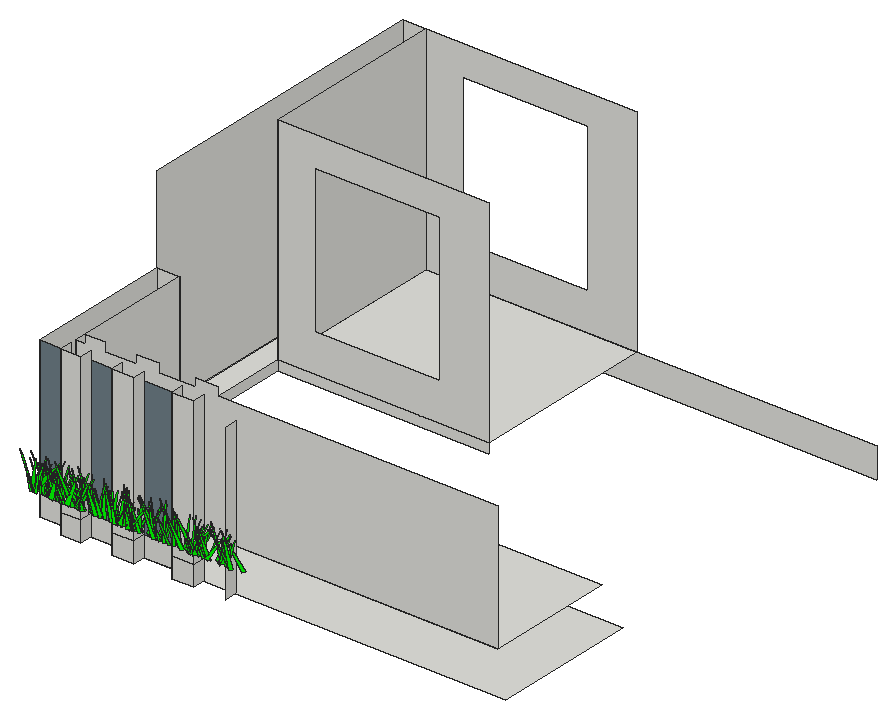
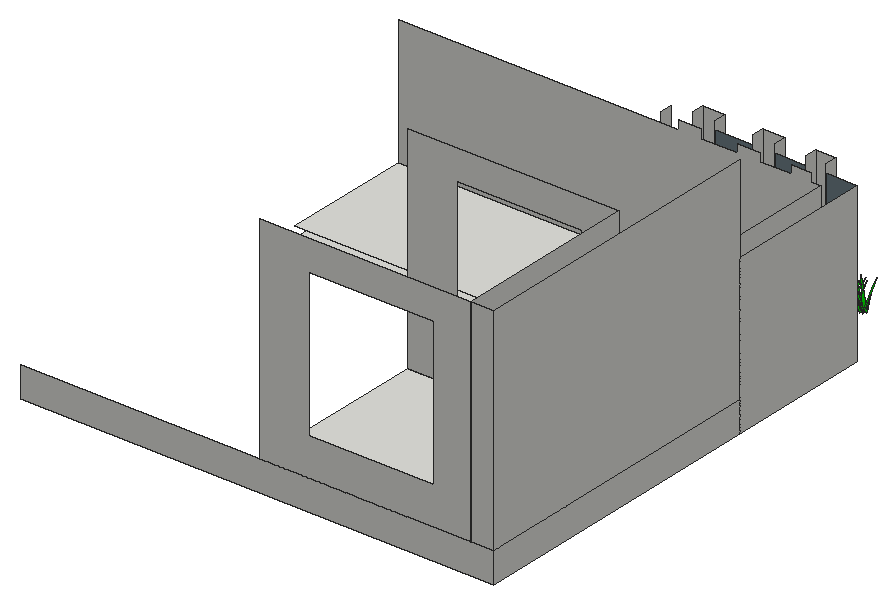
# SketchUp Ruby script. Lengths in inches.
U = 1.inch
M = Sketchup.active_model
def pt(a) = Geom::Point3d.new(a.map { |v| v * U })
def face(e, loops, mat)
  f = e.add_face(loops[0].map { |a| pt(a) })
  loops[1..].each { |l| e.add_face(l.map { |a| pt(a) }).erase! }
  f.material = f.back_material = mat if mat
  f
end
# faces: each face lists its corners as indices into pts; further lists are holes
def faces(e, pts, list, mat = nil) = list.each { |f| face(e, (f[0].is_a?(Array) ? f : [f]).map { |l| l.map { |i| pts[i] } }, mat) }
# xy, xz, yz: faces in a plane at the given z, y or x. An outline is a flat list of corners, or four numbers for a rectangle; further outlines are holes
def ring(l) = l.size == 4 ? [[l[0], l[1]], [l[2], l[1]], [l[2], l[3]], [l[0], l[3]]] : l.each_slice(2).to_a
def flat(e, list, mat, &to3) = list.each { |f| face(e, (f[0].is_a?(Array) ? f : [f]).map { |l| ring(l).map { |u, v| to3.(u, v) } }, mat) }
def xy(e, z, list, mat = nil) = flat(e, list, mat) { |x, y| [x, y, z] }
def xz(e, y, list, mat = nil) = flat(e, list, mat) { |x, z| [x, y, z] }
def yz(e, x, list, mat = nil) = flat(e, list, mat) { |y, z| [x, y, z] }
def lines(e, pts, list) = list.each { |a, b| e.add_line(pt(pts[a]), pt(pts[b])) }
# prism: a flat outline (further loops are holes) pulled along v
def prism(e, loops, v, mat = nil)
  f = face(e, loops, mat); d = Geom::Vector3d.new(v.map { |x| x * U })
  f.pushpull(f.normal.samedirection?(d) ? d.length : -d.length)
end
def box(e, o, s, mat = nil) = prism(e, [[o, [o[0] + s[0], o[1], o[2]], [o[0] + s[0], o[1] + s[1], o[2]], [o[0], o[1] + s[1], o[2]]]], [0, 0, s[2]], mat)
def at(x, y, z, deg = 0) = Geom::Transformation.translation(pt([x, y, z])) * Geom::Transformation.rotation(ORIGIN, Z_AXIS, deg.degrees)
def axes(o, x, y, z) = Geom::Transformation.new([*x, 0, *y, 0, *z, 0, *pt(o).to_a, 1])
def part(name) = M.definitions.add(name)
# library, detail: a bought-in or finely detailed component or shape, given as its bounding box
def library(name, o, s) = part(name).tap { |d| box(d.entities, o, s) }
def detail(e, o, s) = box(e.add_group.entities, o, s)
def put(e, d, t, mat = nil) = e.add_instance(d, t).tap { |i| i.material = mat if mat }
def group(e, t, mat = nil) = e.add_group.tap { |g| g.transformation = t; g.material = mat if mat }.entities
root = M.entities
M.materials.add("[0065_Lime]").color = [0, 255, 0]
M.materials.add("[0111_SlateGray]1").color = [112, 128, 136]
c1 = part("fur_instance\#9")
p = [[0.8125,0,1.79],[0.67,-0.02,1.48],[0,-0.11,0],[0,0.11,0]]
faces(c1.entities,p,[[0,1,2,3]])
xy(root,-11.8125,[[18.06,34.8125,25.54,39.75],[37.97,34.8125,46.56,39.75],[61.07,34.8125,69.9,39.75],[5.71,39.75,187.77,97.05]])
xy(root,0,[[14.21,46.62,179.21,97.05],[5.71,97.05,14.71,217.05],[14.71,144.8,96.96,217.05]])
xz(root,34.8125,[[18.06,-11.8125,25.54,-3.9375],[37.97,-11.8125,46.56,-3.9375],[61.07,-11.8125,69.9,-3.9375],[18.06,-3.9375,25.54,53.25],[37.97,-3.9375,46.56,53.25],
  [61.07,-3.9375,69.9,53.25]])
xz(root,39.75,[[5.71,-11.8125,18.06,-3.9375],[25.54,-11.8125,37.97,-3.9375],[46.56,-11.8125,61.07,-3.9375]])
xz(root,39.75,[[5.71,-3.9375,18.06,49.9375],[25.54,-3.9375,37.97,49.9375],[46.56,-3.9375,61.07,49.9375]],"[0111_SlateGray]1")
xz(root,46.62,[[14.21,0,14.21,49.9375,18.06,49.9375,18.06,53.25,25.54,53.25,25.54,49.9375,37.97,49.9375,37.97,53.25,46.56,53.25,46.56,49.9375,61.07,49.9375,61.07,53.25,69.9,53.25,69.9,49.9375,179.21,49.9375,179.21,0]])
xz(root,97.05,[[5.71,0,14.21,49.9375],[14.21,0,14.71,49.9375]])
xz(root,144.8,[[14.71,-3.9375,96.96,0],[[14.71,0,96.96,84],[29.05,14.85,77.86,72.35]]])
xz(root,217.05,[[5.71,-11.8125,190.59,0],[5.71,0,14.71,84],[[14.71,0,96.96,84],[29.05,14.85,77.86,72.35]]])
yz(root,5.71,[[39.75,-11.8125,97.05,49.9375],[97.05,-11.8125,217.05,0],[97.05,0,217.05,84]])
yz(root,14.21,[[46.62,0,97.05,49.9375]])
yz(root,14.71,[[97.05,-3.9375,144.8,0],[144.8,0,217.05,84]])
yz(root,18.06,[[34.8125,-11.8125,39.75,-3.9375],[34.8125,-3.9375,39.75,53.25]])
yz(root,25.54,[[34.8125,-11.8125,39.75,-3.9375],[34.8125,-3.9375,39.75,53.25]])
yz(root,37.97,[[34.8125,-11.8125,39.75,-3.9375],[34.8125,-3.9375,39.75,53.25]])
yz(root,46.56,[[34.8125,-11.8125,39.75,-3.9375],[34.8125,-3.9375,39.75,53.25]])
yz(root,61.07,[[34.8125,-11.8125,39.75,-3.9375],[34.8125,-3.9375,39.75,53.25]])
yz(root,69.9,[[34.8125,-11.8125,39.75,-3.9375],[34.8125,-3.9375,39.75,53.25]])
yz(root,82.49,[[34.4375,-11.6,39.75,48.65]])
put(root,c1,axes([41.71,32.27,1.48],[4.33195,0.11337,0.46115],[-0.98091,0.53224,1.7119],[-0.10114,-0.30594,3.14903]),"[0065_Lime]")
put(root,c1,axes([10.57,31.76,1.48],[-2.35976,0.59564,0.33042],[-4.03469,-0.33361,1.08708],[1.36172,0.04372,3.79354]),"[0065_Lime]")
put(root,c1,axes([70.67,32.28,1.48],[-4.46444,-0.02377,1.19402],[-0.39835,-0.61279,-1.39426],[1.42292,-0.24613,3.35594]),"[0065_Lime]")
put(root,c1,axes([62.18,32.23,1.48],[-2.3359,-0.64219,0.16019],[4.45315,-0.31213,1.03427],[-1.04619,0.10525,4.04472]),"[0065_Lime]")
put(root,c1,axes([21.09,32.11,1.48],[-5.80841,0.43314,0.64865],[-3.1839,-0.78871,-1.21559],[-0.01972,-0.238,5.20877]),"[0065_Lime]")
put(root,c1,axes([26.06,32.26,1.48],[-0.9862,-0.94635,1.83348],[6.30274,-0.264,-2.32294],[3.27302,0.22323,5.02564]),"[0065_Lime]")
put(root,c1,axes([56.34,31.98,1.48],[-6.05553,0.86304,0.84524],[-6.20995,-0.82043,-1.36562],[-0.48856,-0.26882,6.88155]),"[0065_Lime]")
put(root,c1,axes([8.38,32.48,1.48],[-2.48516,-1.08252,0.9385],[7.4377,-0.38033,-1.66901],[2.31515,0.05984,6.36929]),"[0065_Lime]")
put(root,c1,axes([77.67,32.27,1.48],[-0.79339,-0.86582,1.00223],[6.0769,-0.06133,1.40764],[-1.59867,0.19658,4.85336]),"[0065_Lime]")
put(root,c1,axes([86.75,31.84,1.48],[1.09455,1.06985,1.45468],[-7.35888,0.2268,-1.92578],[-2.64807,-0.18806,5.95294]),"[0065_Lime]")
put(root,c1,axes([46.66,32.18,1.48],[6.04785,0.54472,0.1694],[-3.68145,0.78754,2.10281],[1.23206,-0.32069,5.45175]),"[0065_Lime]")
put(root,c1,axes([48.66,31.79,1.48],[-4.51664,0.20117,0.17695],[-1.1949,-0.57433,1.69918],[0.81797,0.27182,3.45924]),"[0065_Lime]")
put(root,c1,axes([70.49,31.98,1.48],[-4.23495,-0.27981,1.01761],[2.33199,-0.5464,1.38671],[0.30344,0.29406,3.54499]),"[0065_Lime]")
put(root,c1,axes([14.39,32.3,1.48],[6.30222,-0.0403,1.72476],[-0.13396,0.91754,1.04218],[-2.1355,-0.17648,5.02467]),"[0065_Lime]")
put(root,c1,axes([42.49,32,1.48],[-7.14696,-0.2393,0.85014],[1.89816,-0.98349,1.28147],[0.62418,0.25076,5.83719]),"[0065_Lime]")
put(root,c1,axes([48.44,32.31,1.48],[2.36748,-1.00196,2.50606],[6.91986,0.47765,2.07402],[-3.52864,0.26446,5.74866]),"[0065_Lime]")
put(root,c1,axes([71.11,31.84,1.48],[5.66218,0.27971,0.02061],[-1.90106,0.76292,-1.39267],[-0.59075,0.22584,4.67916]),"[0065_Lime]")
put(root,c1,axes([67.18,32.29,1.48],[-6.69229,0.73041,1.14946],[-5.3124,-0.84253,-2.52432],[-0.89145,-0.4625,6.41386]),"[0065_Lime]")
put(root,c1,axes([19.09,32.36,1.48],[-5.70859,-0.071,1.72871],[0.02577,-0.83772,-1.0966],[2.18434,-0.17567,4.53078]),"[0065_Lime]")
put(root,c1,axes([26.21,32.26,1.48],[4.36818,-0.53106,0.3008],[3.76842,0.59646,-0.92106],[0.46817,0.15391,4.60727]),"[0065_Lime]")
put(root,c1,axes([72.5,32.2,1.48],[-0.48281,1.1024,3.21593],[-7.58977,0.22787,-3.37133],[-4.42435,-0.51119,5.43243]),"[0065_Lime]")
put(root,c1,axes([41.125,31.8,1.48],[-5.49042,0.65495,0.23007],[-4.49464,-0.75787,1.32632],[1.2661,0.14975,5.70613]),"[0065_Lime]")
put(root,c1,axes([8.66,32.14,1.48],[-1.90878,0.75502,1.27501],[-5.5526,-0.22615,-1.01257],[-0.70447,-0.26327,4.5263]),"[0065_Lime]")
put(root,c1,axes([50.56,32.2,1.48],[1.17059,-0.77851,2.66973],[5.86519,0.32241,1.4489],[-2.65841,0.36852,4.37225]),"[0065_Lime]")
put(root,c1,axes([86.15,32.24,1.48],[-5.07057,-0.84374,0.464],[5.57861,-0.61623,2.78679],[-2.29325,0.36654,5.75327]),"[0065_Lime]")
put(root,c1,axes([77,32.11,1.48],[3.53661,0.75197,0.25197],[-5.07953,0.45347,1.82348],[1.71241,-0.20791,4.88861]),"[0065_Lime]")
put(root,c1,axes([44.51,32.68,1.48],[8.0949,-0.61479,1.09274],[3.9513,1.13232,1.9803],[-2.30957,-0.21758,7.21798]),"[0065_Lime]")
put(root,c1,axes([16.28,31.9,1.48],[-2.53205,1.04954,1.22543],[-7.17157,-0.40363,1.7795],[2.57404,-0.09214,6.16333]),"[0065_Lime]")
put(root,c1,axes([24.72,32.36,1.48],[-4.40296,-1.10351,1.14391],[7.72191,-0.53272,2.44504],[-2.00544,0.37155,6.90312]),"[0065_Lime]")
put(root,c1,axes([27.31,32.54,1.48],[4.07818,-0.45781,0.32345],[3.06812,0.56339,1.12581],[-1.16594,-0.11876,4.09387]),"[0065_Lime]")
put(root,c1,axes([75.21,32.28,1.48],[-3.60754,0.42954,0.81253],[-3.21576,-0.47983,-0.94684],[-0.03047,-0.21549,3.72785]),"[0065_Lime]")
put(root,c1,axes([17.62,31.99,1.48],[-0.35804,0.98371,0.65762],[-6.75723,-0.01563,-1.65066],[-2.00056,-0.12326,5.45769]),"[0065_Lime]")
put(root,c1,axes([55.91,32.41,1.48],[-6.0947,0.51829,2.52587],[-4.41048,-0.88344,-0.96691],[1.94803,-0.37864,5.71342]),"[0065_Lime]")
put(root,c1,axes([9.09,32.45,1.48],[-8.66687,-0.05355,0.96269],[0.22891,-1.2198,-0.9103],[1.22212,-0.15131,6.9976]),"[0065_Lime]")
put(root,c1,axes([8.875,32.17,1.48],[-0.28933,0.60837,0.81065],[-4.26461,0.0013,-1.03981],[-1.2452,-0.14582,3.37285]),"[0065_Lime]")
put(root,c1,axes([35.36,32.43,1.48],[-0.19215,-0.90348,1.55262],[6.44119,0.04993,1.50107],[-1.86945,0.26491,5.01236]),"[0065_Lime]")
put(root,c1,axes([33.69,32.15,1.48],[-2.52802,1.00452,1.06299],[-7.10416,-0.30065,-1.65832],[-1.53077,-0.26367,5.94065]),"[0065_Lime]")
put(root,c1,axes([60.2,32.17,1.48],[8.32693,-0.25179,3.17868],[2.49423,1.25788,-0.98425],[-3.50156,0.29723,6.85802]),"[0065_Lime]")
put(root,c1,axes([58.74,31.97,1.48],[4.83244,0.23686,0.24352],[-1.38274,0.61427,-1.86589],[-1.00949,0.29248,3.72148]),"[0065_Lime]")
put(root,c1,axes([39.68,32.46,1.48],[-3.09092,-0.88211,2.44051],[6.39484,-0.54194,-1.20515],[2.74154,0.2696,5.56262]),"[0065_Lime]")
put(root,c1,axes([34.46,32.625,1.48],[-1.4279,-0.79185,0.65323],[5.46244,-0.22334,-1.17179],[1.60082,0.05578,4.58115]),"[0065_Lime]")
put(root,c1,axes([46.26,32.09,1.48],[2.60006,1.204,1.91417],[-8.5847,0.42928,-1.33269],[-2.29283,-0.24196,7.16045]),"[0065_Lime]")
put(root,c1,axes([70.95,31.94,1.48],[-7.33494,-0.2064,4.13991],[3.38747,-1.12188,2.09676],[4.07262,0.5614,5.71212]),"[0065_Lime]")
put(root,c1,axes([16.71,32.49,1.48],[5.57475,0.08869,0.24958],[-0.68368,0.76423,1.00416],[-0.15833,-0.17736,4.45169]),"[0065_Lime]")
put(root,c1,axes([20.8,32.42,1.48],[-2.29927,0.8627,1.81718],[-5.70084,-0.10237,-3.14405],[-3.19128,-0.43869,4.30721]),"[0065_Lime]")
put(root,c1,axes([84.91,32.6,1.48],[-2.69463,-0.69854,1.16109],[4.74631,-0.42384,-1.2565],[2.05501,0.06295,4.42454]),"[0065_Lime]")
put(root,c1,axes([11.92,32.18,1.48],[5.61368,0.50199,1.60112],[-3.37027,0.83591,-0.96357],[-2.29736,0.00032,5.32597]),"[0065_Lime]")
put(root,c1,axes([32.76,32.32,1.48],[-0.5471,-0.7816,2.4423],[6.04487,0.0591,1.52967],[-1.84771,0.42476,4.28122]),"[0065_Lime]")
put(root,c1,axes([22.58,31.98,1.48],[0.23893,1.12186,0.13379],[-7.74393,0.02691,1.58977],[1.94921,-0.03062,6.29952]),"[0065_Lime]")
put(root,c1,axes([73.35,32.4,1.48],[3.03492,-0.57134,1.24202],[4.34262,0.39472,-0.93657],[0.07407,0.26852,4.0194]),"[0065_Lime]")
put(root,c1,axes([9.59,32.37,1.48],[5.67515,-0.53055,1.42426],[4.10844,0.78065,-1.08694],[-0.66531,0.29505,5.43696]),"[0065_Lime]")
put(root,c1,axes([68.64,32.49,1.48],[5.8557,1.00358,0.75497],[-6.33522,0.63781,4.10122],[3.42561,-0.53597,6.29415]),"[0065_Lime]")
put(root,c1,axes([27.42,32.25,1.48],[-4.92428,0.00624,0.93904],[0.26433,-0.68529,1.06966],[1.12466,0.18838,3.86017]),"[0065_Lime]")
put(root,c1,axes([82.29,32.05,1.48],[-6.23404,0.04017,2.6623],[1.09701,-0.90438,2.15689],[3.09691,0.40122,4.59515]),"[0065_Lime]")
put(root,c1,axes([40.33,32.51,1.48],[6.78336,0.45066,1.50428],[-3.54224,0.94777,1.05405],[-1.07632,-0.27895,6.01159]),"[0065_Lime]")
put(root,c1,axes([50.05,32.87,1.48],[-2.20132,-1.06917,0.68439],[7.40379,-0.32862,-1.44655],[1.94578,0.04083,6.27845]),"[0065_Lime]")
put(root,c1,axes([81.4,32.5,1.48],[6.18641,0.52059,0.93806],[-3.87465,0.84509,1.19133],[-0.20672,-0.26033,5.7432]),"[0065_Lime]")
put(root,c1,axes([28.46,32.05,1.48],[3.11819,1.14666,1.5579],[-7.31821,0.51243,-2.94697],[-4.08676,-0.04272,6.46584]),"[0065_Lime]")
put(root,c1,axes([19.07,32.59,1.48],[5.55607,0.28488,0.41085],[-2.0865,0.74604,1.33504],[0.1088,-0.24082,4.6219]),"[0065_Lime]")
put(root,c1,axes([20.16,32.06,1.48],[7.88545,0.59374,0.96206],[-3.81,1.09606,-2.00481],[-2.1764,0.23247,6.99533]),"[0065_Lime]")
put(root,c1,axes([84.84,32.8,1.48],[0.39788,-0.77961,0.32687],[5.35276,0.06906,1.20864],[-1.51364,0.0393,4.36009]),"[0065_Lime]")
put(root,c1,axes([39.875,32.24,1.48],[0.49662,0.94788,0.80766],[-6.51635,0.10715,-1.56295],[-2.00672,-0.11338,5.27518]),"[0065_Lime]")
put(root,c1,axes([48.13,32.23,1.48],[-9.02578,-0.00763,1.61642],[0.55865,-1.25562,1.86521],[1.90784,0.33155,7.10094]),"[0065_Lime]")
put(root,c1,axes([12,32.6875,1.48],[-7.21111,0.1503,0.99722],[-1.30849,-1.00092,-1.2055],[0.96688,-0.23364,5.80595]),"[0065_Lime]")
put(root,c1,axes([31.24,32.73,1.48],[6.14218,0.65683,3.38011],[-5.77285,0.91029,1.01329],[-2.40664,-0.50719,6.19607]),"[0065_Lime]")
put(root,c1,axes([44.48,32.89,1.48],[5.48442,-0.63054,0.77681],[4.23978,0.7765,1.315],[-1.75261,-0.09467,5.612]),"[0065_Lime]")
put(root,c1,axes([45.5,32.5,1.48],[2.36492,0.63055,0.9155],[-4.59458,0.29933,0.94439],[0.54127,-0.21411,4.01642]),"[0065_Lime]")
put(root,c1,axes([18.8125,32.86,1.48],[-3.70689,-0.71246,0.80592],[4.85846,-0.53902,-1.18191],[1.75637,-0.01265,4.97032]),"[0065_Lime]")
put(root,c1,axes([27.89,32.82,1.48],[-6.26318,0.55581,0.47408],[-3.55555,-0.7047,-3.39501],[-1.82844,-0.53354,4.97796]),"[0065_Lime]")
put(root,c1,axes([65.875,32.96,1.48],[2.39696,-0.83723,0.15727],[5.82987,0.33533,1.02897],[-1.24487,-0.04166,5.12159]),"[0065_Lime]")
put(root,c1,axes([76.87,32.46,1.48],[-5.01621,-0.15404,0.89577],[1.35495,-0.68963,1.04635],[0.76066,0.21259,4.04336]),"[0065_Lime]")
put(root,c1,axes([26.4,32.98,1.48],[2.39281,-1.20936,0.07474],[8.22641,0.31741,-2.15662],[2.53106,0.11168,6.93874]),"[0065_Lime]")
put(root,c1,axes([18.8125,32.32,1.48],[-7.80871,-0.43793,2.00352],[3.83183,-1.03167,2.32486],[1.0474,0.50934,6.43163]),"[0065_Lime]")
put(root,c1,axes([84.5,32.51,1.48],[-2.20416,0.79755,1.89328],[-5.56408,-0.40627,1.44889],[2.58335,-0.19454,4.73603]),"[0065_Lime]")
put(root,c1,axes([29.04,32.8,1.48],[-3.9563,0.08403,0.55759],[-0.78289,-0.53342,-0.98166],[0.46324,-0.18385,3.10309]),"[0065_Lime]")
put(root,c1,axes([27.77,33.17,1.48],[-5.78996,-0.63039,0.95983],[3.68026,-0.78568,-2.60226],[2.82381,-0.26858,5.35956]),"[0065_Lime]")
put(root,c1,axes([13.18,32.51,1.48],[8.59112,-0.1554,0.71367],[1.2597,1.18711,-1.37132],[-0.6372,0.2516,6.91105]),"[0065_Lime]")
put(root,c1,axes([42.98,32.18,1.48],[-3.79874,1.10106,0.5493],[-7.50833,-0.53908,1.85359],[2.341,0.05769,6.83639]),"[0065_Lime]")
put(root,c1,axes([59.89,32.375,1.48],[3.88751,0.48173,0.10943],[-3.29371,0.53201,-1.06083],[-0.96055,0.12539,4.08046]),"[0065_Lime]")
put(root,c1,axes([9.09,32.9,1.48],[4.19537,-1.13706,0.19997],[7.38244,0.52137,-3.13702],[3.32253,0.27731,6.71777]),"[0065_Lime]")
put(root,c1,axes([25.75,32.67,1.48],[-3.58218,-0.53347,0.47538],[3.6451,-0.43668,1.75267],[-1.21169,0.26349,3.86714]),"[0065_Lime]")
put(root,c1,axes([24.7,32.64,1.48],[2.22182,0.70364,1.15338],[-5.16441,0.27129,1.03649],[0.64383,-0.25214,4.33388]),"[0065_Lime]")
put(root,c1,axes([60.16,32.56,1.48],[1.02602,0.67581,0.65295],[-4.74861,0.11232,1.0414],[1.10698,-0.14454,3.86212]),"[0065_Lime]")
put(root,c1,axes([20.08,32.38,1.48],[6.6181,0.5854,0.02654],[-4.09518,0.91566,-1.12791],[-0.76589,0.16249,6.26024]),"[0065_Lime]")
put(root,c1,axes([77.03,33.01,1.48],[7.49406,0.18358,1.05636],[-1.6533,1.00743,1.89375],[-0.81237,-0.35678,5.89078]),"[0065_Lime]")
put(root,c1,axes([56.11,32.37,1.48],[5.48968,0.52687,0.69805],[-3.29542,0.75261,-1.88757],[-1.98375,0.20777,5.06739]),"[0065_Lime]")
put(root,c1,axes([57.59,32.73,1.48],[-3.24779,1.10312,1.66943],[-7.72135,-0.32466,-2.7503],[-2.49446,-0.43133,6.33967]),"[0065_Lime]")
put(root,c1,axes([35.83,32.63,1.48],[-5.75851,-0.1245,0.91479],[1.15467,-0.79109,1.20152],[0.84647,0.23218,4.58433]),"[0065_Lime]")
put(root,c1,axes([56.9,32.59,1.48],[-8.02857,0.26834,1.681],[-1.64006,-1.15969,1.02056],[2.28644,0.1104,6.6347]),"[0065_Lime]")
put(root,c1,axes([18.77,33.2,1.48],[-5.02117,-0.51669,0.13845],[3.45709,-0.67584,-1.55989],[1.26409,-0.20405,4.816]),"[0065_Lime]")
put(root,c1,axes([23.875,32.79,1.48],[-3.69427,0.46672,0.38877],[-3.2947,-0.48553,-1.18269],[-0.63675,-0.19557,3.86398]),"[0065_Lime]")
put(root,c1,axes([44.625,32.89,1.48],[1.80823,-0.64959,0.78383],[4.5119,0.19488,-1.47503],[1.39355,0.21194,3.75864]),"[0065_Lime]")
put(root,c1,axes([15.59,32.37,1.48],[-7.47838,-0.03194,1.95409],[1.32266,-0.9737,2.8158],[2.01827,0.51975,5.39523]),"[0065_Lime]")
put(root,c1,axes([38.92,33.16,1.48],[-0.50588,-1.20135,1.10077],[8.58901,-0.04603,0.92819],[-1.07402,0.19772,6.9043]),"[0065_Lime]")
put(root,c1,axes([45.625,33.16,1.48],[-3.59451,-0.74516,0.66982],[5.17443,-0.51817,-0.94402],[1.42296,0.00194,5.12483]),"[0065_Lime]")
put(root,c1,axes([33.31,33.46,1.48],[8.59709,-0.49219,0.20453],[3.16898,1.1276,2.79472],[-1.51317,-0.43488,7.01491]),"[0065_Lime]")
put(root,c1,axes([35.08,32.79,1.48],[0.4897,0.7532,1.63464],[-5.4234,0.15175,-1.26802],[-1.8321,-0.24789,4.19054]),"[0065_Lime]")
put(root,c1,axes([43.01,33.09,1.48],[-5.64846,0.20276,0.33224],[-1.48413,-0.72376,-1.89404],[-0.21493,-0.33082,4.3474]),"[0065_Lime]")
put(root,c1,axes([36.7,32.5,1.48],[-5.32999,0.96895,1.02243],[-6.72859,-0.76947,1.22742],[1.96335,-0.00662,6.98212]),"[0065_Lime]")
put(root,c1,axes([43.7,32.25,1.48],[8.12737,0.48314,1.21154],[-2.35777,1.04792,-3.53815],[-2.91226,0.49993,6.24559]),"[0065_Lime]")
put(root,c1,axes([63.88,32.39,1.48],[4.34997,0.76452,0.31956],[-4.84779,0.57418,-2.36882],[-2.50106,0.21678,5.14726]),"[0065_Lime]")
put(root,c1,axes([45.91,32.7,1.48],[-4.8067,0.04359,0.37784],[-0.14201,-0.64225,1.28766],[0.54022,0.21904,3.70032]),"[0065_Lime]")
put(root,c1,axes([71.66,33.25,1.48],[7.24052,-0.41405,0.42168],[2.78677,1.00274,1.33332],[-1.08872,-0.18696,6.21721]),"[0065_Lime]")
put(root,c1,axes([63.77,33.08,1.48],[-5.13989,-0.55362,2.27],[3.77539,-0.81788,-1.02797],[3.00947,0.08051,5.16653]),"[0065_Lime]")
put(root,c1,axes([67.8125,33.18,1.48],[-4.94435,-0.86446,2.31645],[5.87361,-0.79358,-1.62878],[3.38493,0.11432,6.20992]),"[0065_Lime]")
put(root,c1,axes([18.35,33.06,1.48],[7.57991,0.5483,1.74272],[-4.33686,1.04363,1.47797],[-1.00364,-0.36869,6.77525]),"[0065_Lime]")
put(root,c1,axes([55.5,33.33,1.48],[-2.13516,-1.1611,0.15431],[7.97772,-0.28232,1.85342],[-2.16091,0.10499,6.69003]),"[0065_Lime]")
put(root,c1,axes([56.77,33.12,1.48],[3.78406,-0.66099,0.2524],[4.63271,0.51106,-1.10722],[0.87253,0.15315,4.78417]),"[0065_Lime]")
put(root,c1,axes([66.82,32.82,1.48],[-7.68887,-0.25927,1.43989],[2.23032,-1.06553,1.45091],[1.25041,0.30631,6.266]),"[0065_Lime]")
put(root,c1,axes([15.96,32.71,1.48],[-5.27391,0.21477,0.39637],[-1.30333,-0.71082,1.43216],[0.93533,0.22051,4.23055]),"[0065_Lime]")
put(root,c1,axes([81.29,32.82,1.48],[7.91344,0.11754,1.52881],[-0.54188,1.1317,-1.05967],[-1.98458,0.15967,6.38542]),"[0065_Lime]")
put(root,c1,axes([30.47,32.78,1.48],[4.69464,0.07082,0.81509],[-0.13147,0.6365,-1.35201],[-1.11392,0.22333,3.59478]),"[0065_Lime]")
put(root,c1,axes([90.71,32.93,1.48],[-4.54352,1.05371,0.67943],[-6.85792,-0.5196,-3.34082],[-3.14618,-0.38911,6.30102]),"[0065_Lime]")
put(root,c1,axes([19.77,32.93,1.48],[-1.77947,0.74462,0.83746],[-4.888,-0.15761,-2.17606],[-2.29094,-0.2421,3.99241]),"[0065_Lime]")
put(root,c1,axes([11.73,33.17,1.48],[-6.17049,0.0683,1.91773],[-0.94971,-0.90667,-0.93987],[2.21195,-0.19876,4.9462]),"[0065_Lime]")
put(root,c1,axes([74.625,33.11,1.48],[-1.89986,-0.7871,2.11666],[5.7783,-0.36163,-1.0746],[2.18152,0.27239,4.6897]),"[0065_Lime]")
put(root,c1,axes([70.96,33.09,1.48],[7.10829,0.49975,0.67378],[-3.64966,0.96381,1.52097],[0.1212,-0.28687,6.28385]),"[0065_Lime]")
put(root,c1,axes([38.93,33.29,1.48],[-6.76181,-0.4397,1.30886],[2.90033,-0.97383,-1.04862],[1.99219,-0.07466,5.96912]),"[0065_Lime]")
put(root,c1,axes([18.77,33.3,1.48],[7.41066,0.0672,2.33408],[-1.21687,1.0739,1.52026],[-2.64232,-0.3061,5.84603]),"[0065_Lime]")
put(root,c1,axes([53.35,33.17,1.48],[-1.17009,-0.95821,2.5521],[6.55157,-0.34814,-2.39266],[3.66357,0.31655,5.0939]),"[0065_Lime]")
put(root,c1,axes([14.2,33.34,1.48],[-6.39121,-0.36479,0.65226],[2.40574,-0.89362,-1.15032],[1.26294,-0.14385,5.49203]),"[0065_Lime]")
put(root,c1,axes([28.65,32.76,1.48],[-5.70404,0.4752,0.41657],[-3.21484,-0.79265,1.17306],[1.16764,0.13901,5.26478]),"[0065_Lime]")
put(root,c1,axes([24.05,33.24,1.48],[1.33931,-0.75027,0.66252],[5.25012,0.15316,-1.21023],[1.26805,0.1583,4.31097]),"[0065_Lime]")
put(root,c1,axes([8.55,33.43,1.48],[8.40121,0.23854,0.23198],[-1.66226,1.07235,2.88064],[0.44724,-0.49527,6.34881]),"[0065_Lime]")
put(root,c1,axes([58.85,33.22,1.48],[4.14214,-0.60848,0.38906],[4.33009,0.56478,-0.90329],[0.48013,0.15593,4.78986]),"[0065_Lime]")
put(root,c1,axes([35.24,33.29,1.48],[-6.03446,0.10113,0.03256],[-0.70401,-0.81675,-1.32526],[-0.15466,-0.22797,4.76233]),"[0065_Lime]")
put(root,c1,axes([82.4375,33.17,1.48],[-3.45664,-1.03208,2.13096],[7.74051,-0.40528,1.73016],[-0.94572,0.45518,6.37224]),"[0065_Lime]")
put(root,c1,axes([15.28,33.06,1.48],[5.83666,0.96708,1.18425],[-7.02925,0.79147,1.26438],[0.27323,-0.29679,7.2305]),"[0065_Lime]")
put(root,c1,axes([51.07,33.43,1.48],[-4.90874,-0.21428,0.7291],[1.29186,-0.68808,-1.02162],[1.20827,-0.13485,4.05433]),"[0065_Lime]")
put(root,c1,axes([12.25,32.71,1.48],[6.19222,0.8867,0.65042],[-5.89003,0.85854,-2.11787],[-2.40118,0.18066,6.87241]),"[0065_Lime]")
put(root,c1,axes([54.12,33.36,1.48],[2.61139,-1.00302,1.50822],[7.28738,0.30849,-1.47379],[1.13278,0.32767,6.00427]),"[0065_Lime]")
put(root,c1,axes([25.99,32.91,1.48],[-2.58416,1.05177,0.25814],[-7.42356,-0.35315,-0.95473],[-1.00794,-0.09555,6.36984]),"[0065_Lime]")
put(root,c1,axes([80.25,33.43,1.48],[1.49712,-1.0144,1.33934],[7.11997,0.13242,-1.90504],[2.0327,0.28329,5.68639]),"[0065_Lime]")
put(root,c1,axes([57.59,32.96,1.48],[5.50454,0.51801,0.28536],[-3.55977,0.76453,-1.07253],[-1.02039,0.12728,5.28102]),"[0065_Lime]")
put(root,c1,axes([39.9375,33.07,1.48],[-6.19887,0.41103,1.55952],[-2.63647,-0.90941,1.09799],[2.29812,0.0654,5.46625]),"[0065_Lime]")
put(root,c1,axes([26.01,33.15,1.48],[-2.12678,0.67282,0.39211],[-4.7286,-0.27841,-0.96137],[-0.89406,-0.12801,4.15183]),"[0065_Lime]")
put(root,c1,axes([43.71,33.22,1.48],[-5.75919,-0.60299,0.61503],[4.21129,-0.72508,2.27077],[-1.11856,0.37479,5.38264]),"[0065_Lime]")
put(root,c1,axes([74.28,33.39,1.48],[7.06598,0.39333,1.4541],[-3.10549,0.99181,0.99488],[-1.17758,-0.25546,6.10153]),"[0065_Lime]")
put(root,c1,axes([72.97,33.24,1.48],[7.04334,-0.35245,0.49281],[2.57961,0.95573,-1.48934],[0.0629,0.27086,5.8964]),"[0065_Lime]")
put(root,c1,axes([49.53,33.4,1.48],[0.56614,0.6853,1.93449],[-4.98883,-0.06638,1.75395],[2.13358,-0.33705,3.58784]),"[0065_Lime]")
put(root,c1,axes([14.4375,33.37,1.48],[-8.12613,0.5129,0.28942],[-3.65488,-1.12261,-1.23357],[-0.30204,-0.21473,7.14031]),"[0065_Lime]")
put(root,c1,axes([15.68,33.03,1.48],[-5.89197,0.51861,1.8008],[-2.88147,-0.86711,2.12986],[3.1968,0.17426,5.2388]),"[0065_Lime]")
put(root,c1,axes([24.7,33.28,1.48],[2.42988,1.11693,1.5728],[-7.96257,0.25794,2.00122],[1.87568,-0.35195,6.45797]),"[0065_Lime]")
put(root,c1,axes([71.62,33.32,1.48],[5.37342,0.70299,0.21692],[-4.95844,0.73837,1.08407],[0.71683,-0.16227,5.87273]),"[0065_Lime]")
put(root,c1,axes([33.26,33.09,1.48],[6.81787,0.44915,0.25825],[-3.03306,0.93466,-1.49061],[-1.0574,0.21499,5.9408]),"[0065_Lime]")
put(root,c1,axes([63.64,33.4,1.48],[-8.2291,-0.56938,1.08212],[4.25576,-1.12279,1.6165],[0.27808,0.33377,7.28392]),"[0065_Lime]")
put(root,c1,axes([49.66,33.32,1.48],[1.35091,0.82771,0.6718],[-5.72983,0.14915,1.46573],[1.59646,-0.1651,4.69217]),"[0065_Lime]")
put(root,c1,axes([71.96,33.29,1.48],[-3.81909,0.67596,1.54659],[-4.43241,-0.59886,1.52878],[2.66641,-0.02731,4.75648]),"[0065_Lime]")
put(root,c1,axes([39.02,33.28,1.48],[6.17653,-0.48188,0.25417],[2.97264,0.70062,-3.28509],[1.73821,0.51413,4.71493]),"[0065_Lime]")
put(root,c1,axes([74.92,33.29,1.48],[-7.75205,0.16811,0.51486],[-1.04269,-1.07147,1.33564],[0.86295,0.21551,6.2389]),"[0065_Lime]")
put(root,c1,axes([34.6,33.19,1.48],[3.27543,0.44424,0.07278],[-2.80804,0.4168,-1.63655],[-1.45528,0.19562,3.32162]),"[0065_Lime]")
put(root,c1,axes([31.58,33.35,1.48],[-5.51393,1.03003,0.5159],[-7.28067,-0.74778,-1.4575],[-1.06145,-0.22157,7.31734]),"[0065_Lime]")
put(root,c1,axes([16.21,33.36,1.48],[-5.56993,-0.07175,1.15463],[0.98015,-0.75213,1.5623],[1.14671,0.29438,4.273]),"[0065_Lime]")
put(root,c1,axes([47.29,33.1,1.48],[-8.05082,0.50238,0.79081],[-3.08148,-1.08935,2.43316],[2.05716,0.33434,6.73956]),"[0065_Lime]")
put(root,c1,axes([69.25,33.24,1.48],[7.58571,0.43037,0.4326],[-2.82547,1.03674,-1.7798],[-1.2961,0.25874,6.41182]),"[0065_Lime]")
put(root,c1,axes([57.27,33.48,1.48],[7.7513,0.12565,1.62728],[-0.28274,1.08207,-1.90858],[-2.17298,0.30741,6.05305]),"[0065_Lime]")
put(root,c1,axes([47.21,33.4375,1.48],[-6.74458,0.51364,0.39281],[-3.33889,-0.91085,1.9788],[1.5641,0.27047,5.91797]),"[0065_Lime]")
